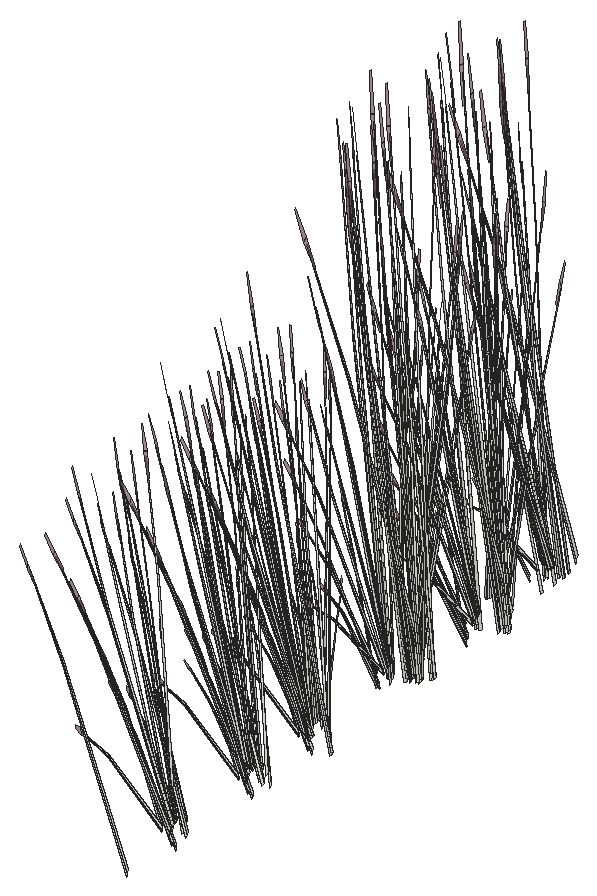
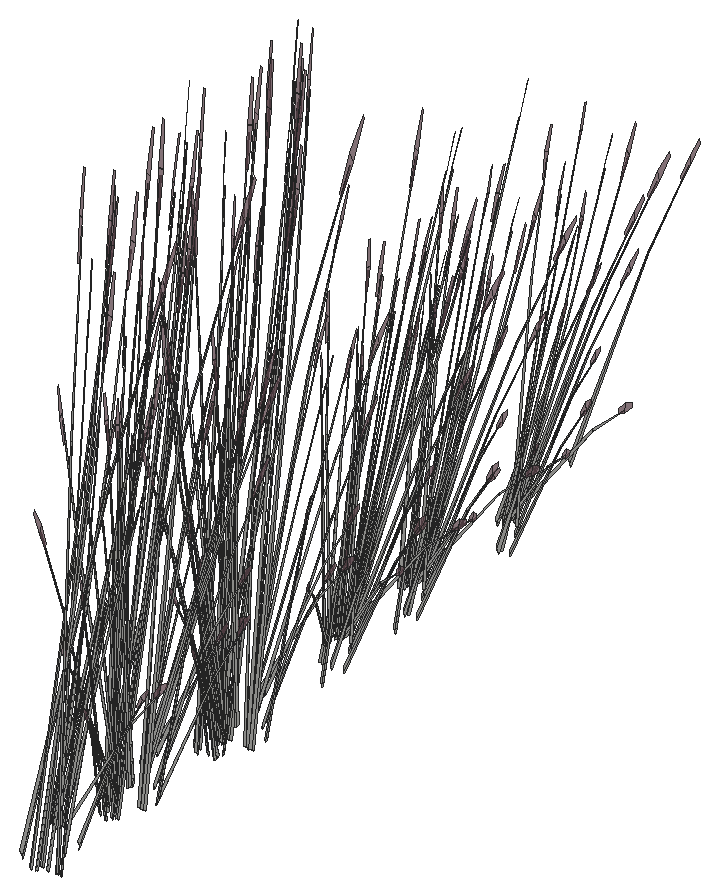
# SketchUp Ruby script. Lengths in inches.
U = 1.inch
M = Sketchup.active_model
def pt(a) = Geom::Point3d.new(a.map { |v| v * U })
def face(e, loops, mat)
  f = e.add_face(loops[0].map { |a| pt(a) })
  loops[1..].each { |l| e.add_face(l.map { |a| pt(a) }).erase! }
  f.material = f.back_material = mat if mat
  f
end
# faces: each face lists its corners as indices into pts; further lists are holes
def faces(e, pts, list, mat = nil) = list.each { |f| face(e, (f[0].is_a?(Array) ? f : [f]).map { |l| l.map { |i| pts[i] } }, mat) }
# xy, xz, yz: faces in a plane at the given z, y or x. An outline is a flat list of corners, or four numbers for a rectangle; further outlines are holes
def ring(l) = l.size == 4 ? [[l[0], l[1]], [l[2], l[1]], [l[2], l[3]], [l[0], l[3]]] : l.each_slice(2).to_a
def flat(e, list, mat, &to3) = list.each { |f| face(e, (f[0].is_a?(Array) ? f : [f]).map { |l| ring(l).map { |u, v| to3.(u, v) } }, mat) }
def xy(e, z, list, mat = nil) = flat(e, list, mat) { |x, y| [x, y, z] }
def xz(e, y, list, mat = nil) = flat(e, list, mat) { |x, z| [x, y, z] }
def yz(e, x, list, mat = nil) = flat(e, list, mat) { |y, z| [x, y, z] }
def lines(e, pts, list) = list.each { |a, b| e.add_line(pt(pts[a]), pt(pts[b])) }
# prism: a flat outline (further loops are holes) pulled along v
def prism(e, loops, v, mat = nil)
  f = face(e, loops, mat); d = Geom::Vector3d.new(v.map { |x| x * U })
  f.pushpull(f.normal.samedirection?(d) ? d.length : -d.length)
end
def box(e, o, s, mat = nil) = prism(e, [[o, [o[0] + s[0], o[1], o[2]], [o[0] + s[0], o[1] + s[1], o[2]], [o[0], o[1] + s[1], o[2]]]], [0, 0, s[2]], mat)
def at(x, y, z, deg = 0) = Geom::Transformation.translation(pt([x, y, z])) * Geom::Transformation.rotation(ORIGIN, Z_AXIS, deg.degrees)
def axes(o, x, y, z) = Geom::Transformation.new([*x, 0, *y, 0, *z, 0, *pt(o).to_a, 1])
def part(name) = M.definitions.add(name)
# library, detail: a bought-in or finely detailed component or shape, given as its bounding box
def library(name, o, s) = part(name).tap { |d| box(d.entities, o, s) }
def detail(e, o, s) = box(e.add_group.entities, o, s)
def put(e, d, t, mat = nil) = e.add_instance(d, t).tap { |i| i.material = mat if mat }
def group(e, t, mat = nil) = e.add_group.tap { |g| g.transformation = t; g.material = mat if mat }.entities
root = M.entities
M.materials.add("LightPink_Translucent").color = [144, 107, 117]
M.materials["LightPink_Translucent"].alpha = 0.75
c1 = part("blade")
p = [[2.15,0.21,22],[0,0.17,0],[0.09,0.45,0],[2.18,0.31,22],[2.29,0.31,22],[0.38,0.45,0],
  [2.48,0.24,33],[2.49,0.24,33],[2.48,0.22,33]]
faces(c1.entities,p,[[0,1,2,3],[4,5,2,3],[6,3,4,7],[8,0,3,6]])
c2 = part("seeds")
p = [[0.3,-0.1,1.38],[-0.01,-0.03,1.59],[-0.01,-0.03,0.03],[0.14,-0.07,-0.07],[0.29,-0.03,3],[0.15,0.01,3.11]]
faces(c2.entities,p,[[0,1,2,3],[1,0,4,5]],"LightPink_Translucent")
c3 = part("blade with seeds")
put(c3.entities,c1,at(0,0,0))
put(c3.entities,c2,axes([2.4,0.25,30.99],[1.5799,-0.05474,1.17369],[-0.12525,1.92788,0.29478],[-0.07173,-0.02425,1.56792]))
put(root,c3,axes([407.8,310.9375,-8.39],[0.21212,-0.01231,1.59586],[-0.14072,0.53355,0.12904],[-0.3023,-0.033,0.68222]))
put(root,c3,axes([406.3,318.6,-8.39],[0.18996,0.09365,1.59586],[-0.39312,0.39287,0.12904],[-0.24502,-0.17723,0.68222]))
put(root,c3,axes([406.26,317.73,-7.61],[-0.11004,-0.00384,1.62908],[-0.35032,0.38367,-0.25764],[-0.18692,-0.07839,0.13065]))
put(root,c3,axes([406.12,319.09,-9.59],[0.09985,0.15133,1.33163],[-0.23008,0.41134,-0.28638],[-0.23625,-0.09832,0.56934]))
put(root,c3,axes([406.53,318.96,-7.36],[-0.51122,-0.01309,-0.66157],[0.03434,-0.5511,0.07984],[-0.21658,-0.05816,0.93586]))
put(root,c3,axes([405.84,318.06,-7.62],[0.03791,0.05424,1.65179],[-0.18278,0.48761,-0.15608],[-0.18511,0.00353,0.29231]))
put(root,c3,axes([406.36,319.07,-7.64],[-0.37135,0.36005,-0.47583],[-0.32522,-0.38035,-0.36857],[-0.18868,-0.05478,0.91046]))
put(root,c3,axes([405.9,319.45,-8.39],[0.21212,-0.01231,1.59586],[-0.14072,0.53355,0.12904],[-0.3023,-0.033,0.68222]))
put(root,c3,axes([405.8125,319.86,-7.59],[0.14449,-0.4956,0.447],[0.47502,0.16947,0.36857],[-0.1868,0.02978,0.92496]))
put(root,c3,axes([405.76,320.11,-10.61],[0.01297,0.08566,1.6421],[-0.26146,0.44735,-0.25086],[-0.18572,-0.02255,0.2797]))
put(root,c3,axes([405.71,319.91,-7.78],[-0.42502,-0.15163,-0.32977],[0.12396,-0.44238,0.42575],[-0.17112,0.04056,0.81462]))
put(root,c3,axes([407.01,319.84,-8.89],[0.14537,-0.07863,1.64882],[0.05013,0.549,0.12904],[-0.31487,0.07285,0.5893]))
put(root,c3,axes([405.44,320.21,-7.61],[-0.08351,0.07057,1.62908],[0.0071,0.51561,-0.25764],[-0.19143,0.06705,0.13065]))
put(root,c3,axes([406,320.14,-7.64],[-0.13855,0.49442,-0.47583],[-0.47502,-0.16947,-0.36857],[-0.19125,0.04534,0.91046]))
put(root,c3,axes([405.98,319.71,-7.3125],[0.25732,0.49218,-0.11324],[-0.45669,0.24187,-0.62851],[-0.19245,0.06494,0.95501]))
put(root,c3,axes([405.99,320.39,-8.39],[0.17745,-0.11497,1.59586],[0.14939,0.53127,0.12904],[-0.27857,0.12007,0.68222]))
put(root,c3,axes([405.43,321.3,-9.59],[0.17773,0.04462,1.33163],[0.11455,0.45576,-0.28638],[-0.24142,0.08531,0.56934]))
put(root,c3,axes([404.52,320.73,-7.62],[0.06527,0.01458,1.65179],[0.20191,0.48025,-0.15608],[-0.1336,0.12605,0.29231]))
put(root,c3,axes([405.0625,322.25,-9.42],[0.21313,-0.24635,1.06958],[0.0841,0.38999,0.78586],[-0.15402,0.06983,0.23558]))
put(root,c3,axes([405.75,329.5,-8.39],[0.18996,0.09365,1.59586],[-0.39312,0.39287,0.12904],[-0.24502,-0.17723,0.68222]))
put(root,c3,axes([405.71,328.63,-7.61],[-0.11004,-0.00384,1.62908],[-0.35032,0.38367,-0.25764],[-0.18692,-0.07839,0.13065]))
put(root,c3,axes([405.63,329.5,-7.26],[0.42234,-0.40113,0.50064],[0.36424,0.42599,0.4128],[-0.19815,-0.07399,1.03595]))
put(root,c3,axes([405.68,329.63,-7.78],[-0.29098,-0.34031,-0.32977],[0.33226,-0.32215,0.42575],[-0.16881,-0.04902,0.81462]))
put(root,c3,axes([405.57,329.99,-9.59],[0.09985,0.15133,1.33163],[-0.23008,0.41134,-0.28638],[-0.23625,-0.09832,0.56934]))
put(root,c3,axes([405.98,329.86,-7.36],[-0.51122,-0.01309,-0.66157],[0.03434,-0.5511,0.07984],[-0.21658,-0.05816,0.93586]))
put(root,c3,axes([405.29,328.96,-7.62],[0.03791,0.05424,1.65179],[-0.18278,0.48761,-0.15608],[-0.18511,0.00353,0.29231]))
put(root,c3,axes([405.81,329.97,-7.64],[-0.37135,0.36005,-0.47583],[-0.32522,-0.38035,-0.36857],[-0.18868,-0.05478,0.91046]))
put(root,c3,axes([404.98,330.44,-9.42],[0.3265,-0.03889,1.06958],[-0.20711,0.3427,0.78586],[-0.16135,-0.05141,0.23558]))
put(root,c3,axes([406.01,329.59,-7.3125],[-0.02738,0.55277,-0.11324],[-0.51847,-0.01511,-0.62851],[-0.19968,-0.0384,0.95501]))
put(root,c3,axes([405.26,330.76,-7.59],[0.14449,-0.4956,0.447],[0.47502,0.16947,0.36857],[-0.1868,0.02978,0.92496]))
put(root,c3,axes([405.23,330.625,-7.6],[-0.18783,-0.37061,0.05988],[0.34252,-0.1814,0.47138],[-0.15099,0.03579,0.71878]))
put(root,c3,axes([405.22,331,-10.61],[0.01297,0.08566,1.6421],[-0.26146,0.44735,-0.25086],[-0.18572,-0.02255,0.2797]))
put(root,c3,axes([405.16,330.81,-7.78],[-0.42502,-0.15163,-0.32977],[0.12396,-0.44238,0.42575],[-0.17112,0.04056,0.81462]))
put(root,c3,axes([406.46,330.74,-8.89],[0.14537,-0.07863,1.64882],[0.05013,0.549,0.12904],[-0.31487,0.07285,0.5893]))
put(root,c3,axes([404.9,331.1,-7.61],[-0.08351,0.07057,1.62908],[0.0071,0.51561,-0.25764],[-0.19143,0.06705,0.13065]))
put(root,c3,axes([405.45,331.04,-7.64],[-0.13855,0.49442,-0.47583],[-0.47502,-0.16947,-0.36857],[-0.19125,0.04534,0.91046]))
put(root,c3,axes([405.43,330.61,-7.3125],[0.25732,0.49218,-0.11324],[-0.45669,0.24187,-0.62851],[-0.19245,0.06494,0.95501]))
put(root,c3,axes([405.375,331.99,-7.59],[-0.12683,-0.50025,0.447],[0.49754,-0.08682,0.36857],[-0.14663,0.11765,0.92496]))
put(root,c3,axes([405.28,331.89,-7.6],[-0.35109,-0.22859,0.05988],[0.2044,-0.32553,0.47138],[-0.11256,0.10524,0.71878]))
put(root,c3,axes([405.4375,331.29,-8.39],[0.17745,-0.11497,1.59586],[0.14939,0.53127,0.12904],[-0.27857,0.12007,0.68222]))
put(root,c3,axes([404.89,332.2,-9.59],[0.17773,0.04462,1.33163],[0.11455,0.45576,-0.28638],[-0.24142,0.08531,0.56934]))
put(root,c3,axes([403.97,331.625,-7.62],[0.06527,0.01458,1.65179],[0.20191,0.48025,-0.15608],[-0.1336,0.12605,0.29231]))
put(root,c3,axes([404.52,333.15,-9.42],[0.21313,-0.24635,1.06958],[0.0841,0.38999,0.78586],[-0.15402,0.06983,0.23558]))
put(root,c3,axes([405.32,332.09,-7.78],[-0.44516,0.07768,-0.32977],[-0.11755,-0.44407,0.42575],[-0.12757,0.11927,0.81462]))
put(root,c3,axes([406.12,338.14,-7.36],[-0.43608,-0.26272,-0.66157],[0.30991,-0.46038,0.07984],[-0.158,-0.15687,0.93586]))
put(root,c3,axes([406.09,331.65,-8.39],[0.12773,-0.16701,1.59586],[0.32252,0.4508,0.12904],[-0.22121,0.20529,0.68222]))
put(root,c3,axes([404.99,338.43,-8.39],[0.18996,0.09365,1.59586],[-0.39312,0.39287,0.12904],[-0.24502,-0.17723,0.68222]))
put(root,c3,axes([405.08,333.4,-10.61],[0.0686,0.0543,1.6421],[0.11632,0.50315,-0.25086],[-0.15204,0.10729,0.2797]))
put(root,c3,axes([405.91,338.15,-7.64],[-0.50465,0.12921,-0.47583],[-0.08828,-0.48932,-0.36857],[-0.13555,-0.14022,0.91046]))
put(root,c3,axes([406.26,337.72,-6.94],[-0.34131,0.52108,-0.12682],[-0.49429,-0.3002,-0.70393],[-0.17182,-0.14722,1.06961]))
put(root,c3,axes([404.96,337.57,-7.61],[-0.11004,-0.00384,1.62908],[-0.35032,0.38367,-0.25764],[-0.18692,-0.07839,0.13065]))
put(root,c3,axes([404.875,338.43,-7.26],[0.42234,-0.40113,0.50064],[0.36424,0.42599,0.4128],[-0.19815,-0.07399,1.03595]))
put(root,c3,axes([405.07,338.43,-7.6],[0.02575,-0.41332,0.05988],[0.38885,0.01133,0.47138],[-0.14895,-0.04325,0.71878]))
put(root,c3,axes([404.92,338.5625,-7.78],[-0.29098,-0.34031,-0.32977],[0.33226,-0.32215,0.42575],[-0.16881,-0.04902,0.81462]))
put(root,c3,axes([404.8125,338.92,-9.59],[0.09985,0.15133,1.33163],[-0.23008,0.41134,-0.28638],[-0.23625,-0.09832,0.56934]))
put(root,c3,axes([405.23,338.79,-7.36],[-0.51122,-0.01309,-0.66157],[0.03434,-0.5511,0.07984],[-0.21658,-0.05816,0.93586]))
put(root,c3,axes([404.53,337.89,-7.62],[0.03791,0.05424,1.65179],[-0.18278,0.48761,-0.15608],[-0.18511,0.00353,0.29231]))
put(root,c3,axes([405.06,338.9,-7.64],[-0.37135,0.36005,-0.47583],[-0.32522,-0.38035,-0.36857],[-0.18868,-0.05478,0.91046]))
put(root,c3,axes([405.33,338.74,-7.3],[0.29098,0.34031,0.32977],[-0.33226,0.32215,-0.42575],[-0.16881,-0.04902,0.81462]))
put(root,c3,axes([404.22,339.38,-9.42],[0.3265,-0.03889,1.06958],[-0.20711,0.3427,0.78586],[-0.16135,-0.05141,0.23558]))
put(root,c3,axes([405.25,338.52,-7.3125],[-0.02738,0.55277,-0.11324],[-0.51847,-0.01511,-0.62851],[-0.19968,-0.0384,0.95501]))
put(root,c3,axes([406.17,340.71,-10.08],[-0.53199,-0.08911,-0.58063],[0.11226,-0.54969,-0.15239],[-0.15876,-0.06661,1.28164]))
put(root,c3,axes([404.5,339.6875,-7.59],[0.14449,-0.4956,0.447],[0.47502,0.16947,0.36857],[-0.1868,0.02978,0.92496]))
put(root,c3,axes([404.47,339.56,-7.6],[-0.18783,-0.37061,0.05988],[0.34252,-0.1814,0.47138],[-0.15099,0.03579,0.71878]))
put(root,c3,axes([404.46,339.9375,-10.61],[0.01297,0.08566,1.6421],[-0.26146,0.44735,-0.25086],[-0.18572,-0.02255,0.2797]))
put(root,c3,axes([404.41,339.74,-7.78],[-0.42502,-0.15163,-0.32977],[0.12396,-0.44238,0.42575],[-0.17112,0.04056,0.81462]))
put(root,c3,axes([404.85,339.69,-7.3],[0.42502,0.15163,0.32977],[-0.12396,0.44238,-0.42575],[-0.17112,0.04056,0.81462]))
put(root,c3,axes([404.14,340.04,-7.61],[-0.08351,0.07057,1.62908],[0.0071,0.51561,-0.25764],[-0.19143,0.06705,0.13065]))
put(root,c3,axes([404.7,339.97,-7.64],[-0.13855,0.49442,-0.47583],[-0.47502,-0.16947,-0.36857],[-0.19125,0.04534,0.91046]))
put(root,c3,axes([404.67,339.55,-7.3125],[0.25732,0.49218,-0.11324],[-0.45669,0.24187,-0.62851],[-0.19245,0.06494,0.95501]))
put(root,c3,axes([404.62,340.92,-7.59],[-0.12683,-0.50025,0.447],[0.49754,-0.08682,0.36857],[-0.14663,0.11765,0.92496]))
put(root,c3,axes([404.52,340.83,-7.6],[-0.35109,-0.22859,0.05988],[0.2044,-0.32553,0.47138],[-0.11256,0.10524,0.71878]))
put(root,c3,axes([403.21,340.56,-7.62],[0.06527,0.01458,1.65179],[0.20191,0.48025,-0.15608],[-0.1336,0.12605,0.29231]))
put(root,c3,axes([403.76,342.08,-9.42],[0.21313,-0.24635,1.06958],[0.0841,0.38999,0.78586],[-0.15402,0.06983,0.23558]))
put(root,c3,axes([404.5625,341.02,-7.78],[-0.44516,0.07768,-0.32977],[-0.11755,-0.44407,0.42575],[-0.12757,0.11927,0.81462]))
put(root,c3,axes([405.33,340.58,-8.39],[0.12773,-0.16701,1.59586],[0.32252,0.4508,0.12904],[-0.22121,0.20529,0.68222]))
put(root,c3,axes([404.93,341.07,-7.64],[0.13138,0.49631,-0.47583],[-0.49754,0.08682,-0.36857],[-0.14258,0.13331,0.91046]))
put(root,c3,axes([404.32,342.34,-10.61],[0.0686,0.0543,1.6421],[0.11632,0.50315,-0.25086],[-0.15204,0.10729,0.2797]))
put(root,c3,axes([405.23,340.99,-8.39],[0.09522,-0.18683,1.59586],[0.39947,0.38663,0.12904],[-0.18021,0.24097,0.68222]))
put(root,c3,axes([404.15,341.96,-7.61],[-0.01271,0.10756,1.62908],[0.36076,0.37419,-0.25764],[-0.09444,0.17695,0.13065]))
put(root,c3,axes([403.1,351.41,-8.39],[0.1169,0.17452,1.59586],[-0.54019,0.14692,0.12904],[-0.12209,-0.27397,0.68222]))
put(root,c3,axes([403.99,350.26,-7.61],[-0.07822,-0.07621,1.62908],[-0.52201,0.04832,-0.25764],[-0.08331,-0.18228,0.13065]))
put(root,c3,axes([402.95,350.95,-9.59],[-0.03097,0.17781,1.33163],[-0.45273,0.14885,-0.28638],[-0.10583,-0.22982,0.56934]))
put(root,c3,axes([403.46,350.01,-7.62],[-0.00954,0.06515,1.65179],[-0.47055,0.23645,-0.15608],[-0.13847,-0.12087,0.29231]))
put(root,c3,axes([403.35,351.16,-7.26],[0.56969,-0.13971,0.50064],[0.09887,0.54803,0.4128],[-0.13398,-0.16152,1.03595]))
put(root,c3,axes([402.79,350.67,-9.42],[0.26677,0.18918,1.06958],[-0.38851,0.11372,0.78586],[-0.08313,-0.14539,0.23558]))
put(root,c3,axes([403.29,351.32,-7.78],[-0.07899,-0.43781,-0.32977],[0.45153,-0.11561,0.42575],[-0.12128,-0.12546,0.81462]))
put(root,c3,axes([403.48,351.28,-7.6],[0.23243,-0.34529,0.05988],[0.331,0.20103,0.47138],[-0.10701,-0.1107,0.71878]))
put(root,c3,axes([404.48,354.64,-8.9],[0.44194,0.21918,1.40854],[-0.43295,0.47219,0.557],[-0.19393,-0.27986,1.18082]))
put(root,c3,axes([403.55,351.68,-7.3],[0.07899,0.43781,0.32977],[-0.45153,0.11561,-0.42575],[-0.12128,-0.12546,0.81462]))
put(root,c3,axes([402.17,353.13,-10.12],[0,-0.54355,-0.46235],[0.57217,0,0],[0,-0.1238,1.46668]))
put(root,c3,axes([402.27,351.51,-10.02],[-0.14753,0.44383,-0.03625],[-0.45406,-0.13653,-0.16435],[-0.06894,-0.07259,0.54209]))
put(root,c3,axes([403.67,353.76,-9.52],[-0.57594,-0.25935,-0.27094],[0.27732,-0.5474,-0.46562],[-0.0181,-0.1344,1.4872]))
put(root,c3,axes([402.03,353.54,-9.79],[-0.63949,0,0],[0,-0.60749,-0.48057],[0,-0.13836,1.52448]))
put(root,c3,axes([402.52,353.38,-9.83],[-0.47569,0.45698,0.2864],[-0.47598,-0.45217,-0.33981],[-0.01661,-0.12977,1.53541]))
put(root,c3,axes([403.8125,354.33,-9.73],[0.13555,-0.64407,-0.21817],[0.64269,0.11227,0.47743],[-0.1123,-0.08895,1.45677]))
put(root,c3,axes([402.42,353.63,-9.69],[0,0.54355,0.46235],[-0.57217,0,0],[0,-0.1238,1.46668]))
put(root,c3,axes([403.77,354.07,-9.94],[-0.30722,-0.45622,-0.41661],[0.46535,-0.32126,0.2005],[-0.09942,-0.05645,1.33761]))
put(root,c3,axes([402.93,355.08,-10.11],[-0.12013,-0.47362,-0.28847],[0.47712,-0.13449,0.28847],[-0.09619,-0.05462,1.29413]))
put(root,c3,axes([404.09,354.33,-9.52],[-0.51635,0.36087,-0.27094],[-0.34336,-0.5099,-0.46562],[-0.1274,-0.05178,1.4872]))
put(root,c3,axes([404.05,354.48,-9.5625],[-0.09866,0.48509,0.13483],[-0.48202,-0.0842,-0.38503],[-0.08772,-0.04981,1.18024]))
put(root,c3,axes([404.67,354.49,-9.7],[-0.49938,-0.43748,-0.23459],[0.42021,-0.49126,0.51337],[-0.13447,0.05118,1.56642]))
put(root,c3,axes([403.36,355.33,-9.69],[0.47863,0.27177,0.46235],[-0.28609,0.48733,0],[-0.10901,-0.0619,1.46668]))
put(root,c3,axes([404.42,354.4,-9.94],[-0.55535,0.03355,-0.41661],[-0.05022,-0.55698,0.2005],[-0.09942,0.05645,1.33761]))
put(root,c3,axes([405.04,355.69,-9.96],[-0.31576,-0.54657,-0.04789],[0.53494,-0.30375,0.48057],[-0.13182,0.05204,1.52373]))
put(root,c3,axes([404.89,355.62,-10.11],[-0.47712,-0.13449,-0.28847],[0.12013,-0.47362,0.28847],[-0.09619,0.05462,1.29413]))
put(root,c3,axes([402.25,354.29,-7.3],[0.44516,-0.07768,0.32977],[0.11755,0.44407,-0.42575],[-0.12757,0.11927,0.81462]))
put(root,c3,axes([401.24,355.55,-6.74],[0.45129,0.14509,-0.06041],[-0.13882,0.44656,-0.27392],[-0.07381,0.0678,0.90349]))
put(root,c3,axes([404.4375,354.72,-10.08],[-0.34446,0.40855,-0.58063],[-0.42791,-0.37046,-0.15239],[-0.13803,0.10191,1.28164]))
put(root,c3,axes([405.01,355.84,-10.12],[-0.47863,0.27177,-0.46235],[-0.28609,-0.48733,0],[-0.10901,0.0619,1.46668]))
put(root,c3,axes([402.85,355.17,-7.3],[0.34603,-0.28618,0.32977],[0.32756,0.32677,-0.42575],[-0.04984,0.16603,0.81462]))
put(root,c3,axes([403.61,362.62,-8.39],[0.1169,0.17452,1.59586],[-0.54019,0.14692,0.12904],[-0.12209,-0.27397,0.68222]))
put(root,c3,axes([405.17,353.59,-9.35],[-0.01397,-0.51177,1.31553],[0.63227,0.13266,0.557],[-0.14954,0.28003,1.24175]))
put(root,c3,axes([402.53,355.43,-7.6],[-0.42027,-0.02533,0.05988],[0.01152,-0.38243,0.47138],[-0.04398,0.14649,0.71878]))
put(root,c3,axes([402.67,355.47,-7.59],[-0.36417,-0.37086,0.447],[0.38674,-0.31985,0.36857],[-0.06718,0.174,0.92496]))
put(root,c3,axes([404.51,361.46,-7.61],[-0.07822,-0.07621,1.62908],[-0.52201,0.04832,-0.25764],[-0.08331,-0.18228,0.13065]))
put(root,c3,axes([403.47,362.16,-9.59],[-0.03097,0.17781,1.33163],[-0.45273,0.14885,-0.28638],[-0.10583,-0.22982,0.56934]))
put(root,c3,axes([402.67,355.58,-7.78],[-0.34603,0.28618,-0.32977],[-0.32756,-0.32677,0.42575],[-0.04984,0.16603,0.81462]))
put(root,c3,axes([402.63,355.25,-6.97],[0.56206,0.02693,-0.12569],[-0.01536,0.50991,-0.69765],[-0.03904,0.19638,1.06006]))
put(root,c3,axes([402.89,356.6875,-9.42],[-0.01324,-0.32319,1.06958],[0.33072,0.23052,0.78586],[-0.06504,0.15405,0.23558]))
put(root,c3,axes([403.97,361.21,-7.62],[-0.00954,0.06515,1.65179],[-0.47055,0.23645,-0.15608],[-0.13847,-0.12087,0.29231]))
put(root,c3,axes([403.87,362.37,-7.26],[0.56969,-0.13971,0.50064],[0.09887,0.54803,0.4128],[-0.13398,-0.16152,1.03595]))
put(root,c3,axes([403.01,355.44,-7.34],[0.3661,0.36521,-0.52818],[-0.38674,0.31985,-0.40911],[-0.0557,0.18556,1.01061]))
put(root,c3,axes([402.61,355.99,-9.37],[0.46459,-0.09625,0.0606],[0.10681,0.38778,-0.80367],[-0.02945,0.1963,0.72038]))
put(root,c3,axes([403.31,361.87,-9.42],[0.26677,0.18918,1.06958],[-0.38851,0.11372,0.78586],[-0.08313,-0.14539,0.23558]))
put(root,c3,axes([403.95,362.875,-7.36],[-0.43608,-0.26272,-0.66157],[0.30991,-0.46038,0.07984],[-0.158,-0.15687,0.93586]))
put(root,c3,axes([403.8,362.53,-7.78],[-0.07899,-0.43781,-0.32977],[0.45153,-0.11561,0.42575],[-0.12128,-0.12546,0.81462]))
put(root,c3,axes([402.9,355.28,-7.03],[-0.01331,0.50278,-0.73435],[-0.56035,-0.03377,0.08862],[-0.05914,0.213,1.03881]))
put(root,c3,axes([401.43,356.6,-7.62],[0.05802,-0.03282,1.65179],[0.47954,0.21828,-0.15608],[-0.01127,0.18175,0.29231]))
put(root,c3,axes([404,362.49,-7.6],[0.23243,-0.34529,0.05988],[0.331,0.20103,0.47138],[-0.10701,-0.1107,0.71878]))
put(root,c3,axes([403.1,362.44,-10.61],[-0.04954,0.0716,1.6421],[-0.50062,0.15438,-0.25086],[-0.12094,-0.14044,0.2797]))
put(root,c3,axes([402.5,356.4,-9.59],[0.16138,-0.08575,1.33163],[0.39845,0.25854,-0.28638],[-0.1186,0.22371,0.56934]))
put(root,c3,axes([403.75,362.89,-7.64],[-0.50465,0.12921,-0.47583],[-0.08828,-0.48932,-0.36857],[-0.13555,-0.14022,0.91046]))
put(root,c3,axes([402.71,355.98,-8.87],[0.01124,-0.2806,1.43727],[0.50537,0.14821,0.19862],[-0.04379,0.29905,0.67868]))
put(root,c3,axes([405,365.85,-8.9],[0.44194,0.21918,1.40854],[-0.43295,0.47219,0.557],[-0.19393,-0.27986,1.18082]))
put(root,c3,axes([404.07,362.88,-7.3],[0.07899,0.43781,0.32977],[-0.45153,0.11561,-0.42575],[-0.12128,-0.12546,0.81462]))
put(root,c3,axes([402.79,362.72,-10.02],[-0.14753,0.44383,-0.03625],[-0.45406,-0.13653,-0.16435],[-0.06894,-0.07259,0.54209]))
put(root,c3,axes([402.54,364.74,-9.79],[-0.63949,0,0],[0,-0.60749,-0.48057],[0,-0.13836,1.52448]))
put(root,c3,axes([403.04,364.58,-9.83],[-0.47569,0.45698,0.2864],[-0.47598,-0.45217,-0.33981],[-0.01661,-0.12977,1.53541]))
put(root,c3,axes([404.33,365.54,-9.73],[0.13555,-0.64407,-0.21817],[0.64269,0.11227,0.47743],[-0.1123,-0.08895,1.45677]))
put(root,c3,axes([403.17,363.48,-7.3],[0.29098,0.34031,0.32977],[-0.33226,0.32215,-0.42575],[-0.16881,-0.04902,0.81462]))
put(root,c3,axes([404.28,365.27,-9.94],[-0.30722,-0.45622,-0.41661],[0.46535,-0.32126,0.2005],[-0.09942,-0.05645,1.33761]))
put(root,c3,axes([403.44,366.29,-10.11],[-0.12013,-0.47362,-0.28847],[0.47712,-0.13449,0.28847],[-0.09619,-0.05462,1.29413]))
put(root,c3,axes([403.31,366.49,-10.12],[-0.47863,-0.27177,-0.46235],[0.28609,-0.48733,0],[-0.10901,-0.0619,1.46668]))
put(root,c3,axes([404.61,365.53,-9.52],[-0.51635,0.36087,-0.27094],[-0.34336,-0.5099,-0.46562],[-0.1274,-0.05178,1.4872]))
put(root,c3,axes([404.5625,365.6875,-9.5625],[-0.09866,0.48509,0.13483],[-0.48202,-0.0842,-0.38503],[-0.08772,-0.04981,1.18024]))
put(root,c3,axes([405.19,365.7,-9.7],[-0.49938,-0.43748,-0.23459],[0.42021,-0.49126,0.51337],[-0.13447,0.05118,1.56642]))
put(root,c3,axes([403.875,366.53,-9.69],[0.47863,0.27177,0.46235],[-0.28609,0.48733,0],[-0.10901,-0.0619,1.46668]))
put(root,c3,axes([403.6,366.82,-9.79],[-0.31974,0.54466,0],[-0.53494,-0.30375,-0.48057],[-0.12184,-0.06918,1.52448]))
put(root,c3,axes([404.9375,365.6,-9.94],[-0.55535,0.03355,-0.41661],[-0.05022,-0.55698,0.2005],[-0.09942,0.05645,1.33761]))
put(root,c3,axes([402.76,365.49,-7.3],[0.44516,-0.07768,0.32977],[0.11755,0.44407,-0.42575],[-0.12757,0.11927,0.81462]))
put(root,c3,axes([401.75,366.75,-6.74],[0.45129,0.14509,-0.06041],[-0.13882,0.44656,-0.27392],[-0.07381,0.0678,0.90349]))
put(root,c3,axes([404.95,365.92,-10.08],[-0.34446,0.40855,-0.58063],[-0.42791,-0.37046,-0.15239],[-0.13803,0.10191,1.28164]))
put(root,c3,axes([402.94,372.1,-7.61],[-0.07822,-0.07621,1.62908],[-0.52201,0.04832,-0.25764],[-0.08331,-0.18228,0.13065]))
put(root,c3,axes([402.53,365.45,-7.3125],[0.47307,0.29971,-0.11324],[-0.27254,0.43404,-0.62851],[-0.13365,0.15087,0.95501]))
put(root,c3,axes([403.49,373.39,-7.36],[-0.24409,-0.44196,-0.66157],[0.50245,-0.2463,0.07984],[-0.05708,-0.21354,0.93586]))
put(root,c3,axes([403.05,366.64,-7.6],[-0.42027,-0.02533,0.05988],[0.01152,-0.38243,0.47138],[-0.04398,0.14649,0.71878]))
put(root,c3,axes([403.18,366.67,-7.59],[-0.36417,-0.37086,0.447],[0.38674,-0.31985,0.36857],[-0.06718,0.174,0.92496]))
put(root,c3,axes([403.3,373.3,-7.64],[-0.50273,-0.13626,-0.47583],[0.17232,-0.46717,-0.36857],[-0.0461,-0.18809,0.91046]))
put(root,c3,axes([402.3,373.01,-7.26],[0.56969,-0.13971,0.50064],[0.09887,0.54803,0.4128],[-0.13398,-0.16152,1.03595]))
put(root,c3,axes([403.73,373.28,-7.3125],[-0.50045,0.25306,-0.11324],[-0.24593,-0.44915,-0.62851],[-0.06603,-0.18927,0.95501]))
put(root,c3,axes([403.18,366.78,-7.78],[-0.34603,0.28618,-0.32977],[-0.32756,-0.32677,0.42575],[-0.04984,0.16603,0.81462]))
put(root,c3,axes([401.74,372.51,-9.42],[0.26677,0.18918,1.06958],[-0.38851,0.11372,0.78586],[-0.08313,-0.14539,0.23558]))
put(root,c3,axes([403.4,367.89,-9.42],[-0.01324,-0.32319,1.06958],[0.33072,0.23052,0.78586],[-0.06504,0.15405,0.23558]))
put(root,c3,axes([402.43,373.13,-7.6],[0.23243,-0.34529,0.05988],[0.331,0.20103,0.47138],[-0.10701,-0.1107,0.71878]))
put(root,c3,axes([402.36,375.05,-10.05],[-0.21003,-0.55738,-0.65031],[0.60499,-0.20074,-0.17068],[-0.02321,-0.18874,1.43544]))
put(root,c3,axes([403.58,373.46,-7.3],[-0.15418,0.41799,0.32977],[-0.44981,-0.12192,-0.42575],[-0.04124,-0.16829,0.81462]))
put(root,c3,axes([403.41,366.48,-7.03],[-0.01331,0.50278,-0.73435],[-0.56035,-0.03377,0.08862],[-0.05914,0.213,1.03881]))
put(root,c3,axes([401.95,367.8,-7.62],[0.05802,-0.03282,1.65179],[0.47954,0.21828,-0.15608],[-0.01127,0.18175,0.29231]))
put(root,c3,axes([402.98,372.79,-10.02],[-0.35341,0.31182,-0.03625],[-0.32382,-0.34152,-0.16435],[-0.0228,-0.09677,0.54209]))
put(root,c3,axes([403.02,367.61,-9.59],[0.16138,-0.08575,1.33163],[0.39845,0.25854,-0.28638],[-0.1186,0.22371,0.56934]))
put(root,c3,axes([403.43,376.49,-8.9],[0.44194,0.21918,1.40854],[-0.43295,0.47219,0.557],[-0.19393,-0.27986,1.18082]))
put(root,c3,axes([401.12,374.97,-10.12],[0,-0.54355,-0.46235],[0.57217,0,0],[0,-0.1238,1.46668]))
put(root,c3,axes([403.23,367.1875,-8.87],[0.01124,-0.2806,1.43727],[0.50537,0.14821,0.19862],[-0.04379,0.29905,0.67868]))
put(root,c3,axes([401.37,374.99,-10.11],[0.35699,-0.33913,-0.28847],[0.35699,0.33913,0.28847],[0,-0.10923,1.29413]))
put(root,c3,axes([402.62,375.6,-9.52],[-0.57594,-0.25935,-0.27094],[0.27732,-0.5474,-0.46562],[-0.0181,-0.1344,1.4872]))
put(root,c3,axes([402.76,376.18,-9.73],[0.13555,-0.64407,-0.21817],[0.64269,0.11227,0.47743],[-0.1123,-0.08895,1.45677]))
put(root,c3,axes([401.37,375.48,-9.69],[0,0.54355,0.46235],[-0.57217,0,0],[0,-0.1238,1.46668]))
put(root,c3,axes([402.72,375.92,-9.94],[-0.30722,-0.45622,-0.41661],[0.46535,-0.32126,0.2005],[-0.09942,-0.05645,1.33761]))
